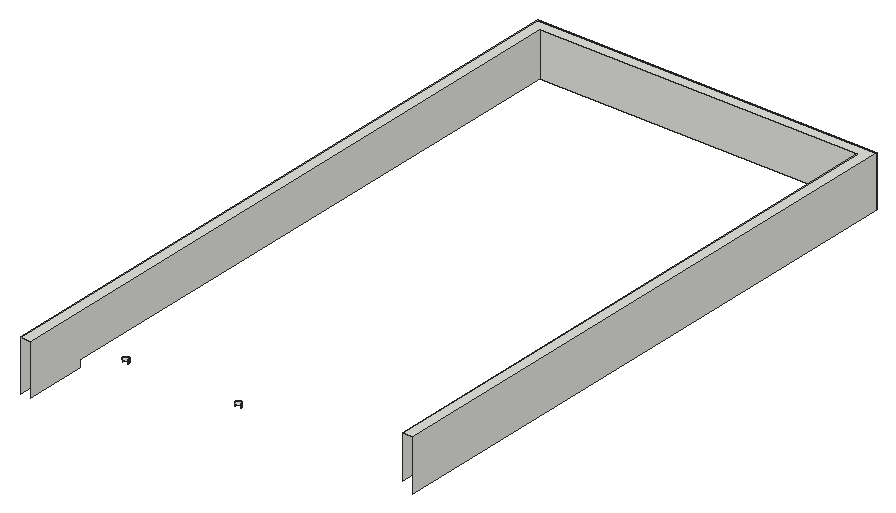
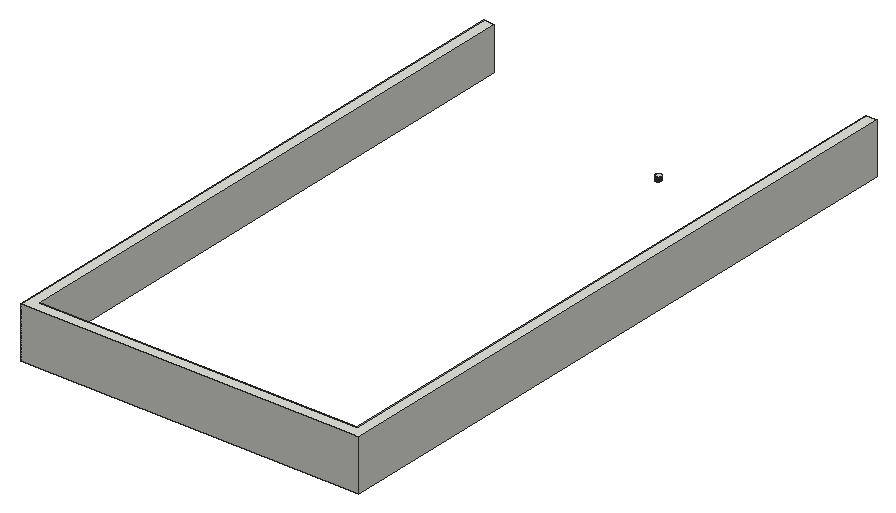
# SketchUp Ruby script. Lengths in inches.
U = 1.inch
M = Sketchup.active_model
def pt(a) = Geom::Point3d.new(a.map { |v| v * U })
def face(e, loops, mat)
  f = e.add_face(loops[0].map { |a| pt(a) })
  loops[1..].each { |l| e.add_face(l.map { |a| pt(a) }).erase! }
  f.material = f.back_material = mat if mat
  f
end
# faces: each face lists its corners as indices into pts; further lists are holes
def faces(e, pts, list, mat = nil) = list.each { |f| face(e, (f[0].is_a?(Array) ? f : [f]).map { |l| l.map { |i| pts[i] } }, mat) }
# xy, xz, yz: faces in a plane at the given z, y or x. An outline is a flat list of corners, or four numbers for a rectangle; further outlines are holes
def ring(l) = l.size == 4 ? [[l[0], l[1]], [l[2], l[1]], [l[2], l[3]], [l[0], l[3]]] : l.each_slice(2).to_a
def flat(e, list, mat, &to3) = list.each { |f| face(e, (f[0].is_a?(Array) ? f : [f]).map { |l| ring(l).map { |u, v| to3.(u, v) } }, mat) }
def xy(e, z, list, mat = nil) = flat(e, list, mat) { |x, y| [x, y, z] }
def xz(e, y, list, mat = nil) = flat(e, list, mat) { |x, z| [x, y, z] }
def yz(e, x, list, mat = nil) = flat(e, list, mat) { |y, z| [x, y, z] }
def lines(e, pts, list) = list.each { |a, b| e.add_line(pt(pts[a]), pt(pts[b])) }
# prism: a flat outline (further loops are holes) pulled along v
def prism(e, loops, v, mat = nil)
  f = face(e, loops, mat); d = Geom::Vector3d.new(v.map { |x| x * U })
  f.pushpull(f.normal.samedirection?(d) ? d.length : -d.length)
end
def box(e, o, s, mat = nil) = prism(e, [[o, [o[0] + s[0], o[1], o[2]], [o[0] + s[0], o[1] + s[1], o[2]], [o[0], o[1] + s[1], o[2]]]], [0, 0, s[2]], mat)
def at(x, y, z, deg = 0) = Geom::Transformation.translation(pt([x, y, z])) * Geom::Transformation.rotation(ORIGIN, Z_AXIS, deg.degrees)
def axes(o, x, y, z) = Geom::Transformation.new([*x, 0, *y, 0, *z, 0, *pt(o).to_a, 1])
def part(name) = M.definitions.add(name)
# library, detail: a bought-in or finely detailed component or shape, given as its bounding box
def library(name, o, s) = part(name).tap { |d| box(d.entities, o, s) }
def detail(e, o, s) = box(e.add_group.entities, o, s)
def put(e, d, t, mat = nil) = e.add_instance(d, t).tap { |i| i.material = mat if mat }
def group(e, t, mat = nil) = e.add_group.tap { |g| g.transformation = t; g.material = mat if mat }.entities
root = M.entities
xy(root,369,[[29.84,216.5,29.76,216.51,29.6875,216.52,29.61,216.53,29.53,216.54,29.45,216.56,29.38,216.58,29.3,216.6,29.23,216.62,29.15,216.65,29.01,216.71,28.9375,216.74,28.87,216.77,28.59,216.93,28.53,216.98,28.47,217.02,28.41,217.07,28.29,217.18,28.23,217.23,28.18,217.29,28.07,217.41,28.02,217.47,27.98,217.53,27.93,217.59,27.77,217.87,27.74,217.9375,27.71,218.01,27.65,218.15,27.62,218.23,27.6,218.3,27.58,218.38,27.56,218.45,27.54,218.53,27.53,218.61,27.52,218.6875,27.51,218.76,27.5,218.84,27.5,219.16,27.51,219.24,27.52,219.3125,27.53,219.39,27.54,219.47,27.56,219.55,27.58,219.62,27.6,219.7,27.62,219.77,27.65,219.85,27.71,219.99,27.74,220.0625,27.77,220.13,27.93,220.41,27.98,220.47,28.02,220.53,28.07,220.59,28.18,220.71,28.23,220.77,28.29,220.82,28.41,220.93,28.47,220.98,28.53,221.02,28.59,221.07,28.87,221.23,28.9375,221.26,29.01,221.29,29.15,221.35,29.23,221.38,29.3,221.4,29.38,221.42,29.45,221.44,29.53,221.46,29.61,221.47,29.6875,221.48,29.76,221.49,29.84,221.5,30.16,221.5,30.24,221.49,30.3125,221.48,30.39,221.47,30.47,221.46,30.55,221.44,30.62,221.42,30.7,221.4,30.77,221.38,30.85,221.35,30.99,221.29,31.0625,221.26,31.13,221.23,31.41,221.07,31.47,221.02,31.53,220.98,31.59,220.93,31.71,220.82,31.77,220.77,31.82,220.71,31.93,220.59,31.98,220.53,32.02,220.47,32.07,220.41,32.23,220.13,32.26,220.0625,32.29,219.99,32.35,219.85,32.38,219.77,32.4,219.7,32.42,219.62,32.44,219.55,32.46,219.47,32.47,219.39,32.48,219.3125,32.49,219.24,32.5,219.16,32.5,218.84,32.49,218.76,32.48,218.6875,32.47,218.61,32.46,218.53,32.44,218.45,32.42,218.38,32.4,218.3,32.38,218.23,32.35,218.15,32.29,218.01,32.26,217.9375,32.23,217.87,32.07,217.59,32.02,217.53,31.98,217.47,31.93,217.41,31.82,217.29,31.77,217.23,31.71,217.18,31.59,217.07,31.53,217.02,31.47,216.98,31.41,216.93,31.13,216.77,31.0625,216.74,30.99,216.71,30.85,216.65,30.77,216.62,30.7,216.6,30.62,216.58,30.55,216.56,30.47,216.54,30.39,216.53,30.3125,216.52,30.24,216.51,30.16,216.5],[123.09,216.5,123.01,216.51,122.9375,216.52,122.86,216.53,122.78,216.54,122.7,216.56,122.63,216.58,122.55,216.6,122.48,216.62,122.4,216.65,122.26,216.71,122.1875,216.74,122.12,216.77,121.84,216.93,121.78,216.98,121.72,217.02,121.66,217.07,121.54,217.18,121.48,217.23,121.43,217.29,121.32,217.41,121.27,217.47,121.23,217.53,121.18,217.59,121.02,217.87,120.99,217.9375,120.96,218.01,120.9,218.15,120.87,218.23,120.85,218.3,120.83,218.38,120.81,218.45,120.79,218.53,120.78,218.61,120.77,218.6875,120.76,218.76,120.75,218.84,120.75,219.16,120.76,219.24,120.77,219.3125,120.78,219.39,120.79,219.47,120.81,219.55,120.83,219.62,120.85,219.7,120.87,219.77,120.9,219.85,120.96,219.99,120.99,220.0625,121.02,220.13,121.18,220.41,121.23,220.47,121.27,220.53,121.32,220.59,121.43,220.71,121.48,220.77,121.54,220.82,121.66,220.93,121.72,220.98,121.78,221.02,121.84,221.07,122.12,221.23,122.1875,221.26,122.26,221.29,122.4,221.35,122.48,221.38,122.55,221.4,122.63,221.42,122.7,221.44,122.78,221.46,122.86,221.47,122.9375,221.48,123.01,221.49,123.09,221.5,123.41,221.5,123.49,221.49,123.5625,221.48,123.64,221.47,123.72,221.46,123.8,221.44,123.87,221.42,123.95,221.4,124.02,221.38,124.1,221.35,124.24,221.29,124.3125,221.26,124.38,221.23,124.66,221.07,124.72,221.02,124.78,220.98,124.84,220.93,124.96,220.82,125.02,220.77,125.07,220.71,125.18,220.59,125.23,220.53,125.27,220.47,125.32,220.41,125.48,220.13,125.51,220.0625,125.54,219.99,125.6,219.85,125.63,219.77,125.65,219.7,125.67,219.62,125.69,219.55,125.71,219.47,125.72,219.39,125.73,219.3125,125.74,219.24,125.75,219.16,125.75,218.84,125.74,218.76,125.73,218.6875,125.72,218.61,125.71,218.53,125.69,218.45,125.67,218.38,125.65,218.3,125.63,218.23,125.6,218.15,125.54,218.01,125.51,217.9375,125.48,217.87,125.32,217.59,125.27,217.53,125.23,217.47,125.18,217.41,125.07,217.29,125.02,217.23,124.96,217.18,124.84,217.07,124.78,217.02,124.72,216.98,124.66,216.93,124.38,216.77,124.3125,216.74,124.24,216.71,124.1,216.65,124.02,216.62,123.95,216.6,123.87,216.58,123.8,216.56,123.72,216.54,123.64,216.53,123.5625,216.52,123.49,216.51,123.41,216.5]])
xy(root,414,[[9,135.92,18,135.92,18,663,281,663,281,192,290,192,290,672,9,672]])
xz(root,221.5,[[29.84,366,29.92,369],[29.92,366,30,369],[30,366,30.08,369],[30.08,366,30.16,369],[123.09,366,123.17,369],
  [123.17,366,123.25,369],[123.25,366,123.33,369],[123.33,366,123.41,369]])
xz(root,663,[[18,378,281,414]])
xz(root,672,[[9,372,290,414]])
yz(root,9,[[135.92,372,672,414]])
yz(root,18,[[135.92,372,186,372,186,378,663,378,663,414,135.92,414]])
yz(root,27.5,[[218.84,366,218.92,369],[218.92,366,219,369],[219,366,219.08,369],[219.08,366,219.16,369]])
yz(root,32.5,[[218.84,366,218.92,369],[218.92,366,219,369],[219,366,219.08,369],[219.08,366,219.16,369]])
yz(root,120.75,[[218.84,366,218.92,369],[218.92,366,219,369],[219,366,219.08,369],[219.08,366,219.16,369]])
yz(root,125.75,[[218.84,366,218.92,369],[218.92,366,219,369],[219,366,219.08,369],[219.08,366,219.16,369]])
yz(root,281,[[192,378,663,414]])
yz(root,290,[[192,372,672,414]])
p = [[27.54,218.53,366],[27.53,218.61,366],[27.53,218.61,369],[27.54,218.53,369],[32.47,218.61,366],[32.46,218.53,366],
  [32.46,218.53,369],[32.47,218.61,369],[120.79,218.53,366],[120.78,218.61,366],[120.78,218.61,369],[120.79,218.53,369],
  [27.52,218.6875,366],[27.52,218.6875,369],[32.48,218.6875,366],[32.48,218.6875,369],[120.77,218.6875,366],[120.77,218.6875,369],
  [125.73,218.6875,366],[125.72,218.61,366],[125.72,218.61,369],[125.73,218.6875,369],[27.51,218.76,366],[27.51,218.76,369],
  [32.49,218.76,366],[32.49,218.76,369],[120.76,218.76,366],[120.76,218.76,369],[125.74,218.76,366],[125.74,218.76,369],
  [27.5,218.84,366],[27.5,218.84,369],[32.5,218.84,366],[32.5,218.84,369],[120.75,218.84,366],[120.75,218.84,369],
  [125.75,218.84,366],[125.75,218.84,369],[27.5,219.16,366],[27.51,219.24,366],[27.51,219.24,369],[27.5,219.16,369],
  [27.52,219.3125,366],[27.52,219.3125,369],[32.49,219.24,366],[32.5,219.16,366],[32.5,219.16,369],[32.49,219.24,369],
  [32.48,219.3125,366],[32.48,219.3125,369],[120.75,219.16,366],[120.76,219.24,366],[120.76,219.24,369],[120.75,219.16,369],
  [120.77,219.3125,366],[120.77,219.3125,369],[125.74,219.24,366],[125.75,219.16,366],[125.75,219.16,369],[125.74,219.24,369],
  [125.73,219.3125,366],[125.73,219.3125,369],[27.53,219.39,366],[27.53,219.39,369],[32.47,219.39,366],[32.47,219.39,369],
  [120.78,219.39,366],[120.78,219.39,369],[125.72,219.39,366],[125.72,219.39,369],[27.54,219.47,366],[27.54,219.47,369],
  [32.46,219.47,366],[32.46,219.47,369],[120.79,219.47,366],[120.79,219.47,369],[125.71,219.47,366],[125.71,219.47,369],
  [27.56,219.55,366],[27.56,219.55,369],[27.58,219.62,366],[27.58,219.62,369],[32.44,219.55,366],[32.44,219.55,369],
  [32.42,219.62,366],[32.42,219.62,369],[120.81,219.55,366],[120.81,219.55,369],[120.83,219.62,366],[120.83,219.62,369],
  [125.69,219.55,366],[125.69,219.55,369],[125.67,219.62,366],[125.67,219.62,369],[27.6,219.7,366],[27.6,219.7,369],
  [32.4,219.7,366],[32.4,219.7,369],[120.85,219.7,366],[120.85,219.7,369],[125.65,219.7,366],[125.65,219.7,369],
  [27.62,219.77,366],[27.62,219.77,369],[32.38,219.77,366],[32.38,219.77,369],[120.87,219.77,366],[120.87,219.77,369],
  [125.63,219.77,366],[125.63,219.77,369],[27.65,219.85,366],[27.65,219.85,369],[27.68,219.92,366],[27.68,219.92,369],
  [32.32,219.92,366],[32.35,219.85,366],[32.35,219.85,369],[32.32,219.92,369],[120.9,219.85,366],[120.9,219.85,369],
  [120.93,219.92,366],[120.93,219.92,369],[125.6,219.85,366],[125.6,219.85,369],[125.57,219.92,366],[125.57,219.92,369],
  [27.71,219.99,366],[27.71,219.99,369],[32.29,219.99,366],[32.29,219.99,369],[120.96,219.99,366],[120.96,219.99,369],
  [125.54,219.99,366],[125.54,219.99,369],[27.74,220.0625,366],[27.74,220.0625,369],[32.26,220.0625,366],[32.26,220.0625,369],
  [120.99,220.0625,366],[120.99,220.0625,369],[125.51,220.0625,366],[125.51,220.0625,369],[27.77,220.13,366],[27.77,220.13,369],
  [27.81,220.2,366],[27.81,220.2,369],[32.23,220.13,366],[32.23,220.13,369],[32.19,220.2,366],[32.19,220.2,369],
  [121.02,220.13,366],[121.02,220.13,369],[121.06,220.2,366],[121.06,220.2,369],[125.44,220.2,366],[125.48,220.13,366],
  [125.48,220.13,369],[125.44,220.2,369],[27.85,220.27,366],[27.85,220.27,369],[32.15,220.27,366],[32.15,220.27,369],
  [121.1,220.27,366],[121.1,220.27,369],[125.4,220.27,366],[125.4,220.27,369],[27.89,220.34,366],[27.89,220.34,369],
  [27.93,220.41,366],[27.93,220.41,369],[32.11,220.34,366],[32.11,220.34,369],[32.07,220.41,366],[32.07,220.41,369],
  [121.14,220.34,366],[121.14,220.34,369],[121.18,220.41,366],[121.18,220.41,369],[125.32,220.41,366],[125.36,220.34,366],
  [125.36,220.34,369],[125.32,220.41,369],[27.98,220.47,366],[27.98,220.47,369],[32.02,220.47,366],[32.02,220.47,369],
  [121.23,220.47,366],[121.23,220.47,369],[125.27,220.47,366],[125.27,220.47,369],[28.02,220.53,366],[28.02,220.53,369],
  [28.07,220.59,366],[28.07,220.59,369],[31.93,220.59,366],[31.98,220.53,366],[31.98,220.53,369],[31.93,220.59,369],
  [121.27,220.53,366],[121.27,220.53,369],[121.32,220.59,366],[121.32,220.59,369],[125.23,220.53,366],[125.23,220.53,369],
  [125.18,220.59,366],[125.18,220.59,369],[28.125,220.65,366],[28.125,220.65,369],[31.875,220.65,366],[31.875,220.65,369],
  [121.375,220.65,366],[121.375,220.65,369],[125.125,220.65,366],[125.125,220.65,369],[28.18,220.71,366],[28.18,220.71,369],
  [28.23,220.77,366],[28.23,220.77,369],[31.82,220.71,366],[31.82,220.71,369],[31.77,220.77,366],[31.77,220.77,369],
  [121.43,220.71,366],[121.43,220.71,369],[121.48,220.77,366],[121.48,220.77,369],[125.02,220.77,366],[125.07,220.71,366],
  [125.07,220.71,369],[125.02,220.77,369],[28.29,220.82,366],[28.29,220.82,369],[28.35,220.875,366],[28.35,220.875,369],
  [31.71,220.82,366],[31.71,220.82,369],[31.65,220.875,366],[31.65,220.875,369],[121.54,220.82,366],[121.54,220.82,369],
  [121.6,220.875,366],[121.6,220.875,369],[124.9,220.875,366],[124.96,220.82,366],[124.96,220.82,369],[124.9,220.875,369],
  [28.41,220.93,366],[28.41,220.93,369],[28.47,220.98,366],[28.47,220.98,369],[31.53,220.98,366],[31.59,220.93,366],
  [31.59,220.93,369],[31.53,220.98,369],[121.66,220.93,366],[121.66,220.93,369],[121.72,220.98,366],[121.72,220.98,369],
  [124.84,220.93,366],[124.84,220.93,369],[124.78,220.98,366],[124.78,220.98,369],[28.53,221.02,366],[28.53,221.02,369],
  [28.59,221.07,366],[28.59,221.07,369],[31.41,221.07,366],[31.47,221.02,366],[31.47,221.02,369],[31.41,221.07,369],
  [121.78,221.02,366],[121.78,221.02,369],[121.84,221.07,366],[121.84,221.07,369],[124.72,221.02,366],[124.72,221.02,369],
  [124.66,221.07,366],[124.66,221.07,369],[28.66,221.11,366],[28.66,221.11,369],[28.73,221.15,366],[28.73,221.15,369],
  [31.34,221.11,366],[31.34,221.11,369],[31.27,221.15,366],[31.27,221.15,369],[121.91,221.11,366],[121.91,221.11,369],
  [121.98,221.15,366],[121.98,221.15,369],[124.52,221.15,366],[124.59,221.11,366],[124.59,221.11,369],[124.52,221.15,369],
  [28.8,221.19,366],[28.8,221.19,369],[28.87,221.23,366],[28.87,221.23,369],[28.9375,221.26,366],[28.9375,221.26,369],
  [31.13,221.23,366],[31.2,221.19,366],[31.2,221.19,369],[31.13,221.23,369],[31.0625,221.26,366],[31.0625,221.26,369],
  [122.05,221.19,366],[122.05,221.19,369],[122.12,221.23,366],[122.12,221.23,369],[122.1875,221.26,366],[122.1875,221.26,369],
  [124.3125,221.26,366],[124.38,221.23,366],[124.38,221.23,369],[124.3125,221.26,369],[124.45,221.19,366],[124.45,221.19,369],
  [29.01,221.29,366],[29.01,221.29,369],[29.08,221.32,366],[29.08,221.32,369],[29.15,221.35,366],[29.15,221.35,369],
  [30.85,221.35,366],[30.92,221.32,366],[30.92,221.32,369],[30.85,221.35,369],[30.99,221.29,366],[30.99,221.29,369],
  [122.26,221.29,366],[122.26,221.29,369],[122.33,221.32,366],[122.33,221.32,369],[122.4,221.35,366],[122.4,221.35,369],
  [124.1,221.35,366],[124.17,221.32,366],[124.17,221.32,369],[124.1,221.35,369],[124.24,221.29,366],[124.24,221.29,369],
  [29.23,221.38,366],[29.23,221.38,369],[29.3,221.4,366],[29.3,221.4,369],[29.38,221.42,366],[29.38,221.42,369],
  [29.45,221.44,366],[29.45,221.44,369],[29.53,221.46,366],[29.53,221.46,369],[30.55,221.44,366],[30.62,221.42,366],
  [30.62,221.42,369],[30.55,221.44,369],[30.47,221.46,366],[30.47,221.46,369],[30.7,221.4,366],[30.7,221.4,369],
  [30.77,221.38,366],[30.77,221.38,369],[122.48,221.38,366],[122.48,221.38,369],[122.55,221.4,366],[122.55,221.4,369],
  [122.63,221.42,366],[122.63,221.42,369],[122.7,221.44,366],[122.7,221.44,369],[122.78,221.46,366],[122.78,221.46,369],
  [123.72,221.46,366],[123.8,221.44,366],[123.8,221.44,369],[123.72,221.46,369],[123.87,221.42,366],[123.87,221.42,369],
  [123.95,221.4,366],[124.02,221.38,366],[124.02,221.38,369],[123.95,221.4,369],[29.61,221.47,366],[29.61,221.47,369],
  [29.6875,221.48,366],[29.6875,221.48,369],[29.76,221.49,366],[29.76,221.49,369],[29.84,221.5,366],[29.84,221.5,369],
  [30.24,221.49,366],[30.3125,221.48,366],[30.3125,221.48,369],[30.24,221.49,369],[30.16,221.5,366],[30.16,221.5,369],
  [30.39,221.47,366],[30.39,221.47,369],[122.86,221.47,366],[122.86,221.47,369],[122.9375,221.48,366],[122.9375,221.48,369],
  [123.01,221.49,366],[123.01,221.49,369],[123.09,221.5,366],[123.09,221.5,369],[123.41,221.5,366],[123.49,221.49,366],
  [123.49,221.49,369],[123.41,221.5,369],[123.5625,221.48,366],[123.5625,221.48,369],[123.64,221.47,366],[123.64,221.47,369]]
faces(root,p,[[0,1,2,3],[4,5,6,7],[8,9,10,11],[1,12,13,2],[14,4,7,15],[9,16,17,10],[18,19,20,21],[12,22,23,13],
  [24,14,15,25],[16,26,27,17],[28,18,21,29],[22,30,31,23],[32,24,25,33],[26,34,35,27],[36,28,29,37],[38,39,40,41],
  [39,42,43,40],[44,45,46,47],[48,44,47,49],[50,51,52,53],[51,54,55,52],[56,57,58,59],[60,56,59,61],[42,62,63,43],
  [64,48,49,65],[54,66,67,55],[68,60,61,69],[62,70,71,63],[72,64,65,73],[66,74,75,67],[76,68,69,77],[70,78,79,71],
  [78,80,81,79],[82,72,73,83],[84,82,83,85],[74,86,87,75],[86,88,89,87],[90,76,77,91],[92,90,91,93],[80,94,95,81],
  [96,84,85,97],[88,98,99,89],[100,92,93,101],[94,102,103,95],[104,96,97,105],[98,106,107,99],[108,100,101,109],[102,110,111,103],
  [110,112,113,111],[114,115,116,117],[115,104,105,116],[106,118,119,107],[118,120,121,119],[122,108,109,123],[124,122,123,125],[112,126,127,113],
  [128,114,117,129],[120,130,131,121],[132,124,125,133],[126,134,135,127],[136,128,129,137],[130,138,139,131],[140,132,133,141],[134,142,143,135],
  [142,144,145,143],[146,136,137,147],[148,146,147,149],[138,150,151,139],[150,152,153,151],[154,155,156,157],[155,140,141,156],[144,158,159,145],
  [160,148,149,161],[152,162,163,153],[164,154,157,165],[158,166,167,159],[166,168,169,167],[170,160,161,171],[172,170,171,173],[162,174,175,163],
  [174,176,177,175],[178,179,180,181],[179,164,165,180],[168,182,183,169],[184,172,173,185],[176,186,187,177],[188,178,181,189],[182,190,191,183],
  [190,192,193,191],[194,195,196,197],[195,184,185,196],[186,198,199,187],[198,200,201,199],[202,188,189,203],[204,202,203,205],[192,206,207,193],
  [208,194,197,209],[200,210,211,201],[212,204,205,213],[206,214,215,207],[214,216,217,215],[218,208,209,219],[220,218,219,221],[210,222,223,211],
  [222,224,225,223],[226,227,228,229],[227,212,213,228],[216,230,231,217],[230,232,233,231],[234,220,221,235],[236,234,235,237],[224,238,239,225],
  [238,240,241,239],[242,243,244,245],[243,226,229,244],[232,246,247,233],[246,248,249,247],[250,251,252,253],[251,236,237,252],[240,254,255,241],
  [254,256,257,255],[258,242,245,259],[260,258,259,261],[248,262,263,249],[262,264,265,263],[266,267,268,269],[267,250,253,268],[256,270,271,257],
  [270,272,273,271],[274,260,261,275],[276,274,275,277],[264,278,279,265],[278,280,281,279],[282,266,269,283],[284,282,283,285],[272,286,287,273],
  [286,288,289,287],[290,291,292,293],[291,276,277,292],[280,294,295,281],[294,296,297,295],[296,298,299,297],[300,301,302,303],[304,300,303,305],
  [301,284,285,302],[288,306,307,289],[306,308,309,307],[308,310,311,309],[312,313,314,315],[313,316,317,314],[316,290,293,317],[298,318,319,299],
  [318,320,321,319],[320,322,323,321],[324,325,326,327],[325,328,329,326],[328,304,305,329],[310,330,331,311],[330,332,333,331],[332,334,335,333],
  [336,337,338,339],[340,312,315,341],[337,340,341,338],[322,342,343,323],[342,344,345,343],[344,346,347,345],[346,348,349,347],[348,350,351,349],
  [352,353,354,355],[356,352,355,357],[353,358,359,354],[358,360,361,359],[360,324,327,361],[334,362,363,335],[362,364,365,363],[364,366,367,365],
  [366,368,369,367],[368,370,371,369],[372,373,374,375],[373,376,377,374],[378,379,380,381],[376,378,381,377],[379,336,339,380],[350,382,383,351],
  [382,384,385,383],[384,386,387,385],[386,388,389,387],[390,391,392,393],[394,390,393,395],[391,396,397,392],[396,356,357,397],[370,398,399,371],
  [398,400,401,399],[400,402,403,401],[402,404,405,403],[406,407,408,409],[407,410,411,408],[412,372,375,413],[410,412,413,411]])
